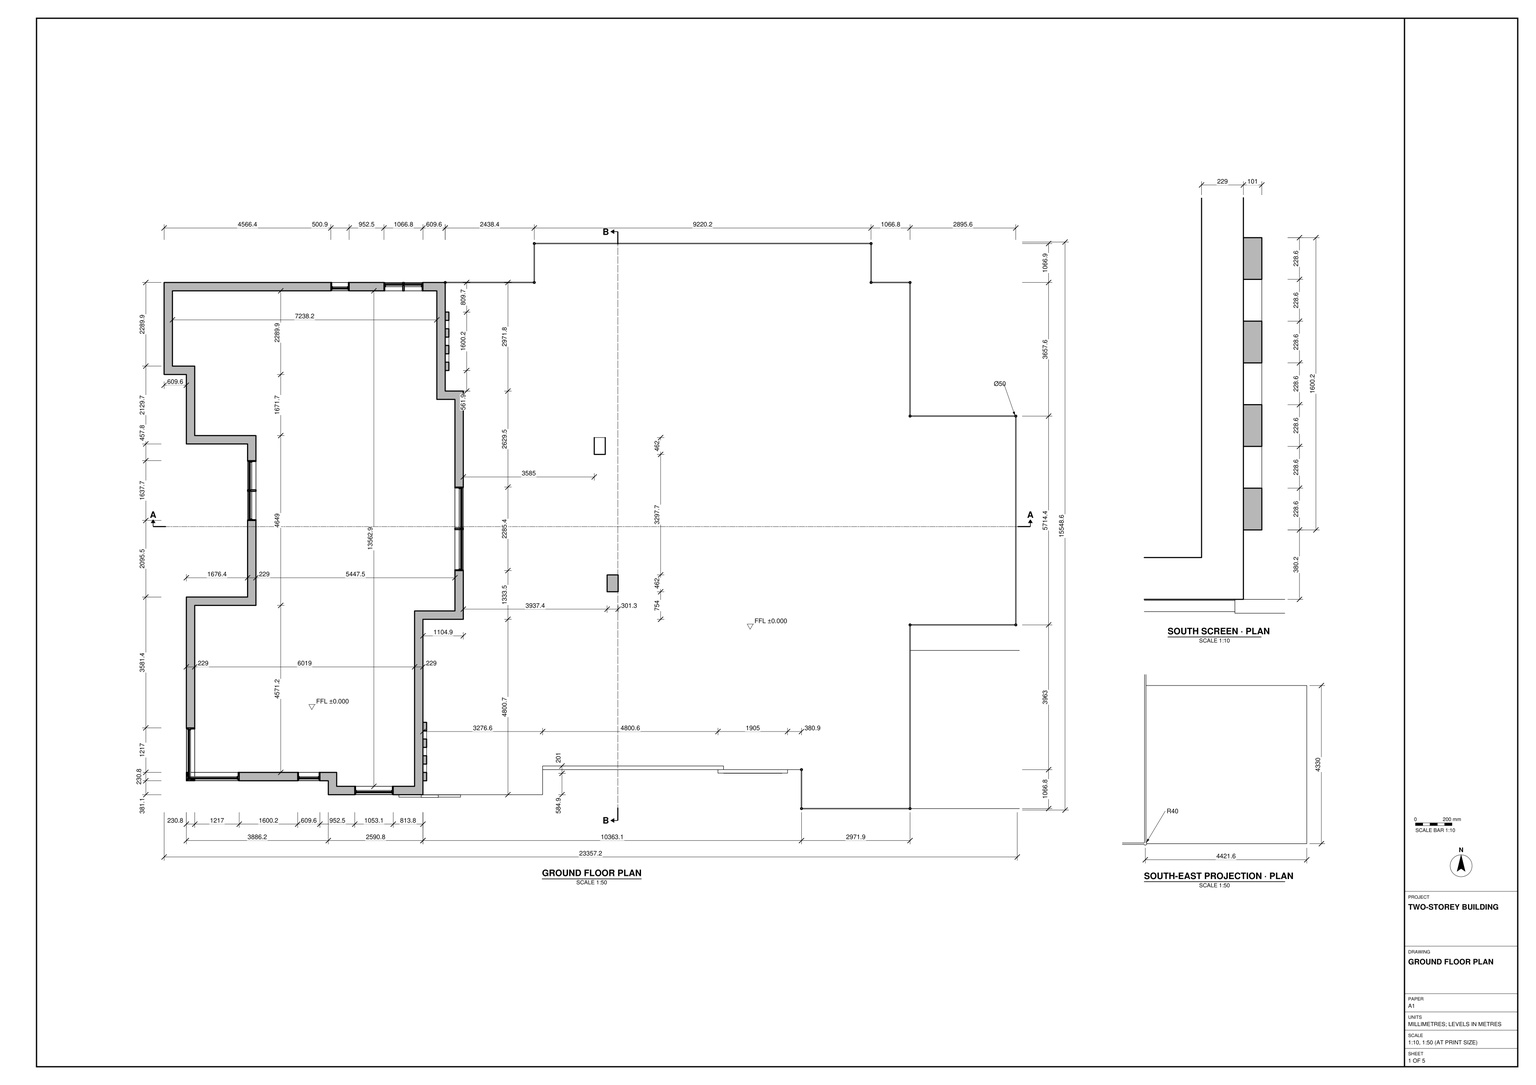
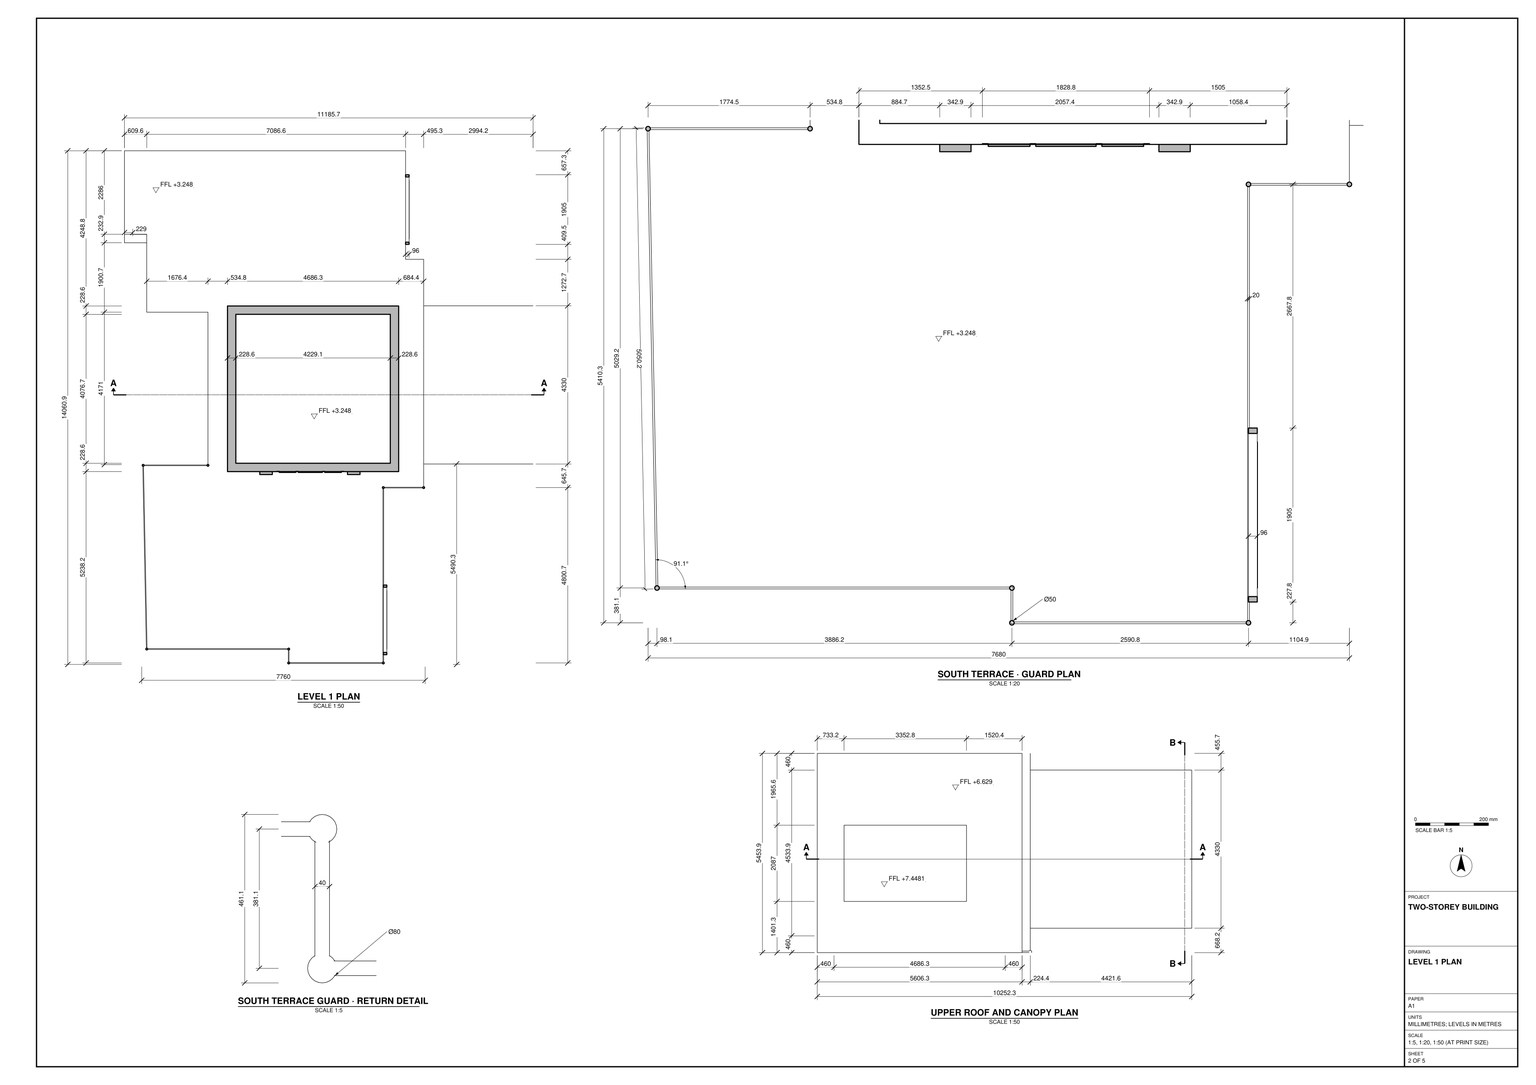
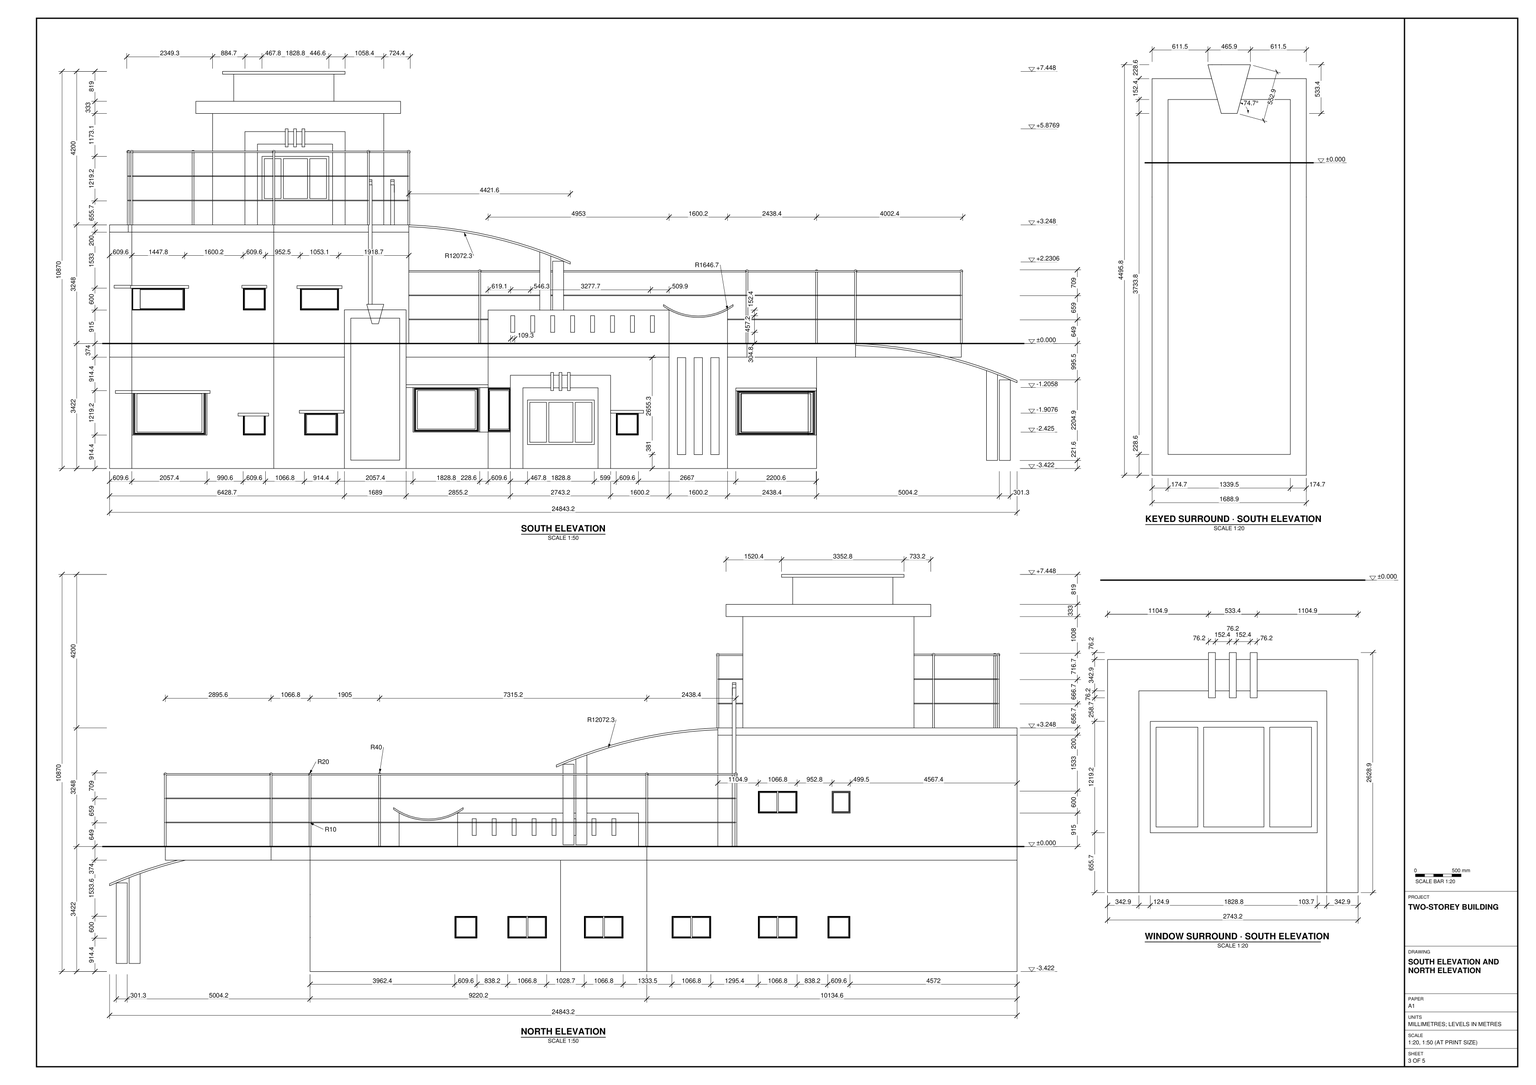
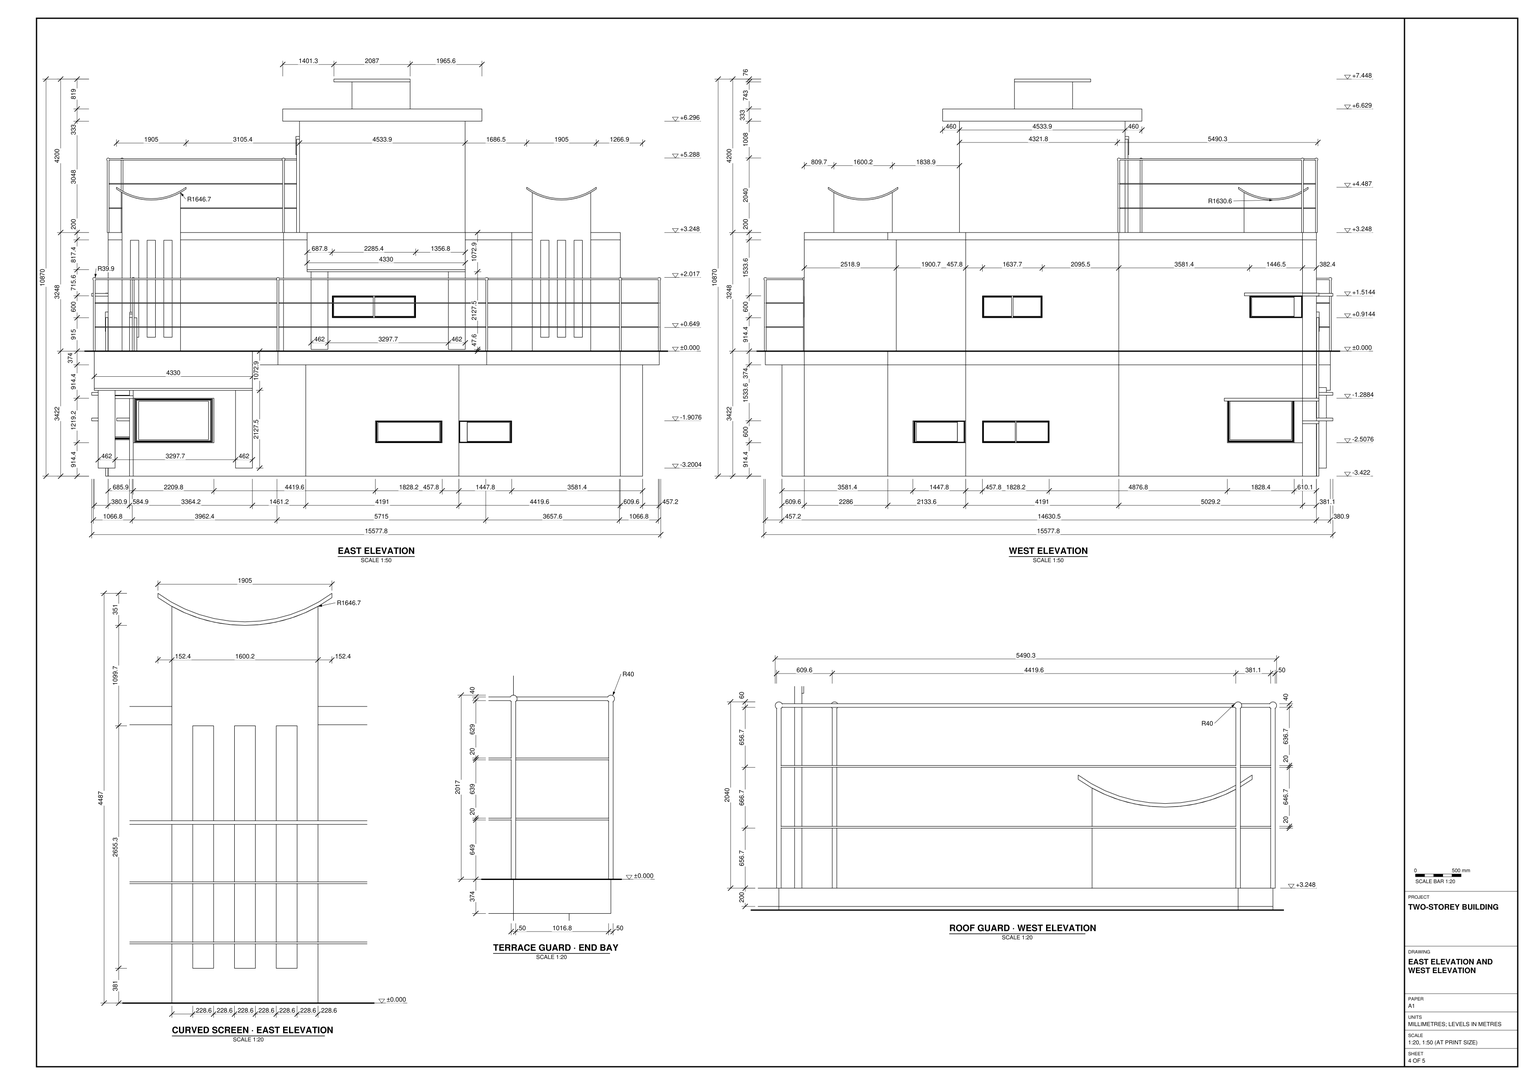
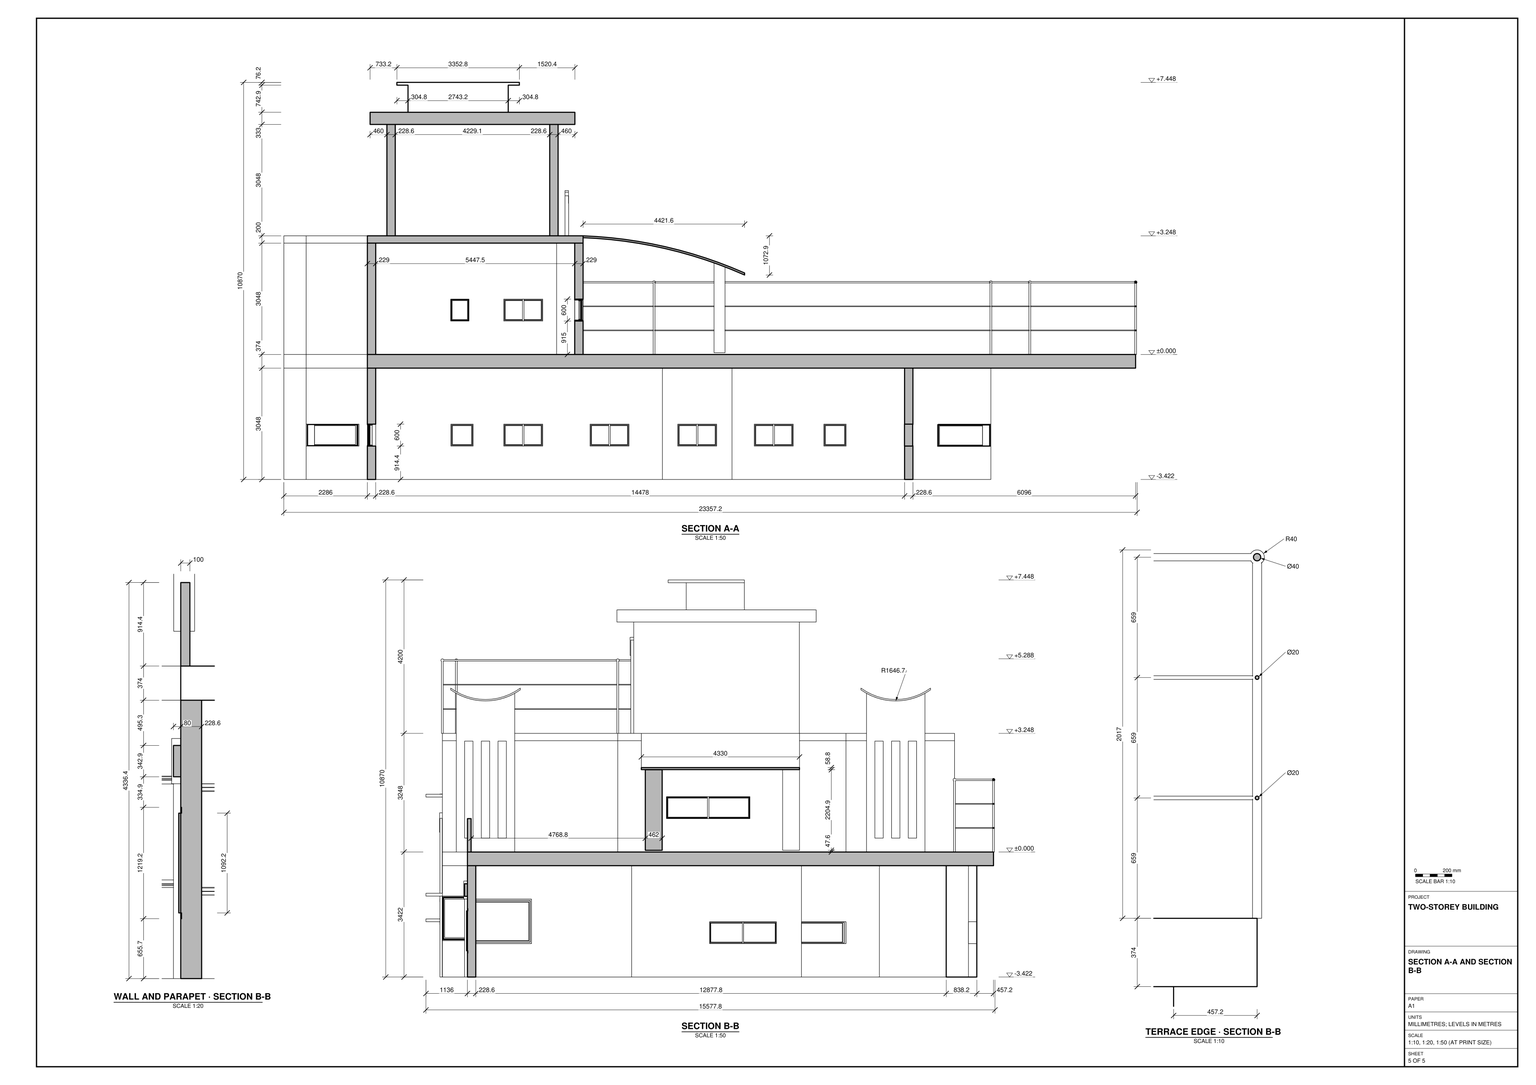
Build the building shown in task_files/diagram_01.pdf in SketchUp. Work in millimetres. The overall extents, including roof edges and canopy projections, are 24843.2 mm along X, 15577.7 mm along Y and 10870.1 mm along Z. Set the ground-floor datum at 0 mm and Level 1 at +3248 mm. Include the part of the building below the ground-floor datum shown in the elevations.

Trace the stepped ground-floor enclosure on the west side of the plan, using the drawn wall thickness of 229 mm. Above it, form the smaller rectangular enclosure with 228.6 mm walls. Follow the slab outlines so that the terraces retain their recesses and projecting corners. Model the terrace guards with horizontal rails, posts and the south return. Give the upper enclosure its overhanging flat roof and smaller raised cap. Follow the elevation profiles for the curved canopies and place their supports as drawn.

Set the window openings and frame divisions from the elevations. Include the tall keyed surround, the framed south windows and the vertical screen detail. Keep shell elements and each furniture or joinery piece shown in separate groups or components, and use components for repeated parts. Decor and loose items may be any suitable library components. Save one SketchUp model as output_files/two_storey_building_stepped_terraces_and_curved_canopies.skp.

# SketchUp Ruby script. Lengths in millimetres.
U = 1.mm
M = Sketchup.active_model
def pt(a) = Geom::Point3d.new(a.map { |v| v * U })
def face(e, loops, mat)
  f = e.add_face(loops[0].map { |a| pt(a) })
  loops[1..].each { |l| e.add_face(l.map { |a| pt(a) }).erase! }
  f.material = f.back_material = mat if mat
  f
end
# faces: each face lists its corners as indices into pts; further lists are holes
def faces(e, pts, list, mat = nil) = list.each { |f| face(e, (f[0].is_a?(Array) ? f : [f]).map { |l| l.map { |i| pts[i] } }, mat) }
# xy, xz, yz: faces in a plane at the given z, y or x. An outline is a flat list of corners, or four numbers for a rectangle; further outlines are holes
def ring(l) = l.size == 4 ? [[l[0], l[1]], [l[2], l[1]], [l[2], l[3]], [l[0], l[3]]] : l.each_slice(2).to_a
def flat(e, list, mat, &to3) = list.each { |f| face(e, (f[0].is_a?(Array) ? f : [f]).map { |l| ring(l).map { |u, v| to3.(u, v) } }, mat) }
def xy(e, z, list, mat = nil) = flat(e, list, mat) { |x, y| [x, y, z] }
def xz(e, y, list, mat = nil) = flat(e, list, mat) { |x, z| [x, y, z] }
def yz(e, x, list, mat = nil) = flat(e, list, mat) { |y, z| [x, y, z] }
def lines(e, pts, list) = list.each { |a, b| e.add_line(pt(pts[a]), pt(pts[b])) }
# prism: a flat outline (further loops are holes) pulled along v
def prism(e, loops, v, mat = nil)
  f = face(e, loops, mat); d = Geom::Vector3d.new(v.map { |x| x * U })
  f.pushpull(f.normal.samedirection?(d) ? d.length : -d.length)
end
def box(e, o, s, mat = nil) = prism(e, [[o, [o[0] + s[0], o[1], o[2]], [o[0] + s[0], o[1] + s[1], o[2]], [o[0], o[1] + s[1], o[2]]]], [0, 0, s[2]], mat)
def at(x, y, z, deg = 0) = Geom::Transformation.translation(pt([x, y, z])) * Geom::Transformation.rotation(ORIGIN, Z_AXIS, deg.degrees)
def axes(o, x, y, z) = Geom::Transformation.new([*x, 0, *y, 0, *z, 0, *pt(o).to_a, 1])
def part(name) = M.definitions.add(name)
# library, detail: a bought-in or finely detailed component or shape, given as its bounding box
def library(name, o, s) = part(name).tap { |d| box(d.entities, o, s) }
def detail(e, o, s) = box(e.add_group.entities, o, s)
def put(e, d, t, mat = nil) = e.add_instance(d, t).tap { |i| i.material = mat if mat }
def group(e, t, mat = nil) = e.add_group.tap { |g| g.transformation = t; g.material = mat if mat }.entities
root = M.entities
M.materials.add("[0012_Bisque]").color = [255, 228, 196]
M.materials.add("[Stone Marble]").color = [143, 138, 136]
M.materials.add("[Wood Cherry Original]").color = [152, 86, 42]
c1 = part("Difference\#1")
xy(c1.entities,0,[[[4495.8,0,4495.8,381.1,609.6,381.1,609.6,5410.3,2286,5410.3,2286,9601.3,609.6,9601.3,609.6,11734.9,0,11734.9,0,14020.9,10134.6,14020.9,10134.6,14630.5,12496.8,14630.5,12496.8,14020.9,19354.8,14020.9,19354.8,9601.3,17221.2,9601.3,17221.2,5410.3,19354.8,5410.3,19354.8,685.9,10363.2,685.9,10363.2,0],[4724.4,228.6,10134.6,228.6,10134.6,914.5,19126.2,914.5,19126.2,5181.7,16992.6,5181.7,16992.6,9829.9,19126.2,9829.9,19126.2,13792.3,12268.2,13792.3,12268.2,14401.9,10363.2,14401.9,10363.2,13792.3,228.6,13792.3,228.6,11963.5,838.2,11963.5,838.2,9829.9,2514.6,9829.9,2514.6,5181.7,838.2,5181.7,838.2,609.7,4724.4,609.7]]])
xy(c1.entities,914.4,[[5334,0,6248.4,228.6],[609.6,381.1,2667,381.1,2667,609.7,838.2,609.7,838.2,2438.5,609.6,2438.5],[3657.6,381.1,4267.2,609.7],[13868.4,685.9,14478,914.5],[17145,685.9,19354.8,685.9,19354.8,2895.7,19126.2,2895.7,19126.2,914.5,17145,914.5],
  [2286,7315.3,2514.6,9143.5],[16992.6,7315.3,17221.2,9143.5],[609.6,9601.3,2057.4,9601.3,2057.4,9829.9,838.2,9829.9,838.2,11049.1,609.6,11049.1],[17907,9601.3,19354.8,9601.3,19354.8,11049.1,19126.2,11049.1,19126.2,9829.9,17907,9829.9],[4572,13792.3,5181.6,14020.9],
  [6019.8,13792.3,7086.6,14020.9],[8382,13792.3,9448.8,14020.9],[12877.8,13792.3,13944.6,14020.9],[14782.8,13792.3,15392.4,14020.9],[10782.3,14401.9,11849.1,14630.5]])
xy(c1.entities,997,[[8305.8,0,10363.2,0,10363.2,685.9,10972.8,685.9,10972.8,914.5,10134.6,914.5,10134.6,228.6,8305.8,228.6]])
xy(c1.entities,1514.4,[[5334,0,6248.4,228.6],[3657.6,381.1,4267.2,609.7],[13868.4,685.9,14478,914.5],[2286,7315.3,2514.6,9143.5],[16992.6,7315.3,17221.2,9143.5],
  [609.6,9601.3,609.6,11049.1,838.2,11049.1,838.2,9829.9,2057.4,9829.9,2057.4,9601.3],[17907,9601.3,17907,9829.9,19126.2,9829.9,19126.2,11049.1,19354.8,11049.1,19354.8,9601.3],[4572,13792.3,5181.6,14020.9],[6019.8,13792.3,7086.6,14020.9],[8382,13792.3,9448.8,14020.9],
  [12877.8,13792.3,13944.6,14020.9],[14782.8,13792.3,15392.4,14020.9],[10782.3,14401.9,11849.1,14630.5]])
xy(c1.entities,2133.6,[[609.6,381.1,609.6,2438.5,838.2,2438.5,838.2,609.7,2667,609.7,2667,381.1],[17145,685.9,17145,914.5,19126.2,914.5,19126.2,2895.7,19354.8,2895.7,19354.8,685.9]])
xy(c1.entities,2216.2,[[8305.8,0,8305.8,228.6,10134.6,228.6,10134.6,914.5,10972.8,914.5,10972.8,685.9,10363.2,685.9,10363.2,0]])
xy(c1.entities,3048,[[[4495.8,0,10363.2,0,10363.2,685.9,19354.8,685.9,19354.8,5410.3,17221.2,5410.3,17221.2,9601.3,19354.8,9601.3,19354.8,14020.9,12496.8,14020.9,12496.8,14630.5,10134.6,14630.5,10134.6,14020.9,0,14020.9,0,11734.9,609.6,11734.9,609.6,9601.3,2286,9601.3,2286,5410.3,609.6,5410.3,609.6,381.1,4495.8,381.1],[4724.4,228.6,4724.4,609.7,838.2,609.7,838.2,5181.7,2514.6,5181.7,2514.6,9829.9,838.2,9829.9,838.2,11963.5,228.6,11963.5,228.6,13792.3,10363.2,13792.3,10363.2,14401.9,12268.2,14401.9,12268.2,13792.3,19126.2,13792.3,19126.2,9829.9,16992.6,9829.9,16992.6,5181.7,19126.2,5181.7,19126.2,914.5,10134.6,914.5,10134.6,228.6]]])
xz(c1.entities,0,[[[4495.8,0,10363.2,0,10363.2,997,8305.8,997,8305.8,2216.2,10363.2,2216.2,10363.2,3048,4495.8,3048],[5334,914.4,6248.4,1514.4]]])
xz(c1.entities,228.6,[[[4724.4,0,4724.4,3048,10134.6,3048,10134.6,2216.2,8305.8,2216.2,8305.8,997,10134.6,997,10134.6,0],[5334,914.4,6248.4,1514.4]]])
xz(c1.entities,381.1,[[[609.6,0,4495.8,0,4495.8,3048,609.6,3048,609.6,2133.6,2667,2133.6,2667,914.4,609.6,914.4],[3657.6,914.4,4267.2,1514.4]]])
xz(c1.entities,609.7,[[[838.2,0,838.2,914.4,2667,914.4,2667,2133.6,838.2,2133.6,838.2,3048,4724.4,3048,4724.4,0],[3657.6,914.4,4267.2,1514.4]]])
xz(c1.entities,685.9,[[[10363.2,0,19354.8,0,19354.8,914.4,17145,914.4,17145,2133.6,19354.8,2133.6,19354.8,3048,10363.2,3048,10363.2,2216.2,10972.8,2216.2,10972.8,997,10363.2,997],[13868.4,914.4,14478,1514.4]]])
xz(c1.entities,914.5,[[[10134.6,0,10134.6,997,10972.8,997,10972.8,2216.2,10134.6,2216.2,10134.6,3048,19126.2,3048,19126.2,2133.6,17145,2133.6,17145,914.4,19126.2,914.4,19126.2,0],[13868.4,914.4,14478,1514.4]]])
xz(c1.entities,2438.5,[[609.6,914.4,838.2,2133.6]])
xz(c1.entities,2895.7,[[19126.2,914.4,19354.8,2133.6]])
xz(c1.entities,5181.7,[[838.2,0,2514.6,3048],[16992.6,0,19126.2,3048]])
xz(c1.entities,5410.3,[[609.6,0,2286,3048],[17221.2,0,19354.8,3048]])
xz(c1.entities,7315.3,[[2286,914.4,2514.6,1514.4],[16992.6,914.4,17221.2,1514.4]])
xz(c1.entities,9143.5,[[2286,914.4,2514.6,1514.4],[16992.6,914.4,17221.2,1514.4]])
xz(c1.entities,9601.3,[[609.6,0,2286,0,2286,3048,609.6,3048,609.6,1514.4,2057.4,1514.4,2057.4,914.4,609.6,914.4],[17221.2,0,19354.8,0,19354.8,914.4,17907,914.4,17907,1514.4,19354.8,1514.4,19354.8,3048,17221.2,3048]])
xz(c1.entities,9829.9,[[838.2,0,838.2,914.4,2057.4,914.4,2057.4,1514.4,838.2,1514.4,838.2,3048,2514.6,3048,2514.6,0],[16992.6,0,16992.6,3048,19126.2,3048,19126.2,1514.4,17907,1514.4,17907,914.4,19126.2,914.4,19126.2,0]])
xz(c1.entities,11049.1,[[609.6,914.4,838.2,1514.4],[19126.2,914.4,19354.8,1514.4]])
xz(c1.entities,11734.9,[[0,0,609.6,3048]])
xz(c1.entities,11963.5,[[228.6,0,838.2,3048]])
xz(c1.entities,13792.3,[[[228.6,0,10363.2,3048],[8382,914.4,9448.8,1514.4],[6019.8,914.4,7086.6,1514.4],[4572,914.4,5181.6,1514.4]],[[12268.2,0,19126.2,3048],[12877.8,914.4,13944.6,1514.4],[14782.8,914.4,15392.4,1514.4]]])
xz(c1.entities,14020.9,[[[0,0,10134.6,3048],[8382,914.4,9448.8,1514.4],[6019.8,914.4,7086.6,1514.4],[4572,914.4,5181.6,1514.4]],[[12496.8,0,19354.8,3048],[12877.8,914.4,13944.6,1514.4],[14782.8,914.4,15392.4,1514.4]]])
xz(c1.entities,14401.9,[[[10363.2,0,12268.2,3048],[10782.3,914.4,11849.1,1514.4]]])
xz(c1.entities,14630.5,[[[10134.6,0,12496.8,3048],[10782.3,914.4,11849.1,1514.4]]])
yz(c1.entities,0,[[11734.9,0,14020.9,3048]])
yz(c1.entities,228.6,[[11963.5,0,13792.3,3048]])
yz(c1.entities,609.6,[[381.1,0,381.1,914.4,2438.5,914.4,2438.5,2133.6,381.1,2133.6,381.1,3048,5410.3,3048,5410.3,0],[9601.3,0,9601.3,914.4,11049.1,914.4,11049.1,1514.4,9601.3,1514.4,9601.3,3048,11734.9,3048,11734.9,0]])
yz(c1.entities,838.2,[[609.7,0,5181.7,0,5181.7,3048,609.7,3048,609.7,2133.6,2438.5,2133.6,2438.5,914.4,609.7,914.4],[9829.9,0,11963.5,0,11963.5,3048,9829.9,3048,9829.9,1514.4,11049.1,1514.4,11049.1,914.4,9829.9,914.4]])
yz(c1.entities,2057.4,[[9601.3,914.4,9829.9,1514.4]])
yz(c1.entities,2286,[[[5410.3,0,9601.3,3048],[7315.3,914.4,9143.5,1514.4]]])
yz(c1.entities,2514.6,[[[5181.7,0,9829.9,3048],[7315.3,914.4,9143.5,1514.4]]])
yz(c1.entities,2667,[[381.1,914.4,609.7,2133.6]])
yz(c1.entities,3657.6,[[381.1,914.4,609.7,1514.4]])
yz(c1.entities,4267.2,[[381.1,914.4,609.7,1514.4]])
yz(c1.entities,4495.8,[[0,0,381.1,3048]])
yz(c1.entities,4572,[[13792.3,914.4,14020.9,1514.4]])
yz(c1.entities,4724.4,[[228.6,0,609.7,3048]])
yz(c1.entities,5181.6,[[13792.3,914.4,14020.9,1514.4]])
yz(c1.entities,5334,[[0,914.4,228.6,1514.4]])
yz(c1.entities,6019.8,[[13792.3,914.4,14020.9,1514.4]])
yz(c1.entities,6248.4,[[0,914.4,228.6,1514.4]])
yz(c1.entities,7086.6,[[13792.3,914.4,14020.9,1514.4]])
yz(c1.entities,8305.8,[[0,997,228.6,2216.2]])
yz(c1.entities,8382,[[13792.3,914.4,14020.9,1514.4]])
yz(c1.entities,9448.8,[[13792.3,914.4,14020.9,1514.4]])
yz(c1.entities,10134.6,[[228.6,0,914.5,997],[14020.9,0,14630.5,3048],[228.6,2216.2,914.5,3048]])
yz(c1.entities,10363.2,[[0,0,685.9,997],[13792.3,0,14401.9,3048],[0,2216.2,685.9,3048]])
yz(c1.entities,10782.3,[[14401.9,914.4,14630.5,1514.4]])
yz(c1.entities,10972.8,[[685.9,997,914.5,2216.2]])
yz(c1.entities,11849.1,[[14401.9,914.4,14630.5,1514.4]])
yz(c1.entities,12268.2,[[13792.3,0,14401.9,3048]])
yz(c1.entities,12496.8,[[14020.9,0,14630.5,3048]])
yz(c1.entities,12877.8,[[13792.3,914.4,14020.9,1514.4]])
yz(c1.entities,13868.4,[[685.9,914.4,914.5,1514.4]])
yz(c1.entities,13944.6,[[13792.3,914.4,14020.9,1514.4]])
yz(c1.entities,14478,[[685.9,914.4,914.5,1514.4]])
yz(c1.entities,14782.8,[[13792.3,914.4,14020.9,1514.4]])
yz(c1.entities,15392.4,[[13792.3,914.4,14020.9,1514.4]])
yz(c1.entities,16992.6,[[[5181.7,0,9829.9,3048],[7315.3,914.4,9143.5,1514.4]]])
yz(c1.entities,17145,[[685.9,914.4,914.5,2133.6]])
yz(c1.entities,17221.2,[[[5410.3,0,9601.3,3048],[7315.3,914.4,9143.5,1514.4]]])
yz(c1.entities,17907,[[9601.3,914.4,9829.9,1514.4]])
yz(c1.entities,19126.2,[[914.5,0,914.5,914.4,2895.7,914.4,2895.7,2133.6,914.5,2133.6,914.5,3048,5181.7,3048,5181.7,0],[9829.9,0,9829.9,914.4,11049.1,914.4,11049.1,1514.4,9829.9,1514.4,9829.9,3048,13792.3,3048,13792.3,0]])
yz(c1.entities,19354.8,[[685.9,0,5410.3,0,5410.3,3048,685.9,3048,685.9,2133.6,2895.7,2133.6,2895.7,914.4,685.9,914.4],[9601.3,0,14020.9,0,14020.9,3048,9601.3,3048,9601.3,1514.4,11049.1,1514.4,11049.1,914.4,9601.3,914.4]])
c2 = part("Group\#19")
box(c2.entities,[-87,0,0],[1590,450,77])
c3 = part("Group\#20")
g1 = group(c3.entities,at(0,-450,0))
box(g1,[0,0,0],[2141,450,77])
c4 = library("Group\#35",[0,0,0],[609.6,230.8,600])
c5 = part("Difference\#7")
xy(c5.entities,0,[[[4495.8,0,4495.8,381.1,609.6,381.1,609.6,5410.3,2286,5410.3,2286,9601.3,609.6,9601.3,609.6,11502,0,11502,0,14020.9,7696.2,14020.9,7696.2,11049.1,8191.5,11049.1,8191.5,4800.7,7086.6,4800.7,7086.6,0],[4724.8,229,6857.6,229,6857.6,5029.7,7962.5,5029.7,7962.5,10820.1,7467.2,10820.1,7467.2,13791.9,229,13791.9,229,11731,838.6,11731,838.6,9830.3,2515,9830.3,2515,5181.3,838.6,5181.3,838.6,610.1,4724.8,610.1]]])
xy(c5.entities,914.4,[[609.6,381.1,2057.4,381.1,2057.4,610.1,838.6,610.1,838.6,1828.9,609.6,1828.9]])
xy(c5.entities,915,[[5219.7,0,6272.8,229],[3657.6,381.1,4267.2,610.1],[7962.5,6134.2,8191.5,8419.6],[2286,7505.8,2515,9143.5],[4566.4,13791.9,5067.3,14020.9],
  [6019.8,13791.9,7086.6,14020.9]])
xy(c5.entities,1514.4,[[609.6,381.1,609.6,1828.9,838.6,1828.9,838.6,610.1,2057.4,610.1,2057.4,381.1]])
xy(c5.entities,1515,[[5219.7,0,6272.8,229],[3657.6,381.1,4267.2,610.1],[7962.5,6134.2,8191.5,8419.6],[2286,7505.8,2515,9143.5],[4566.4,13791.9,5067.3,14020.9],
  [6019.8,13791.9,7086.6,14020.9]])
xy(c5.entities,3048,[[[4495.8,0,7086.6,0,7086.6,4800.7,8191.5,4800.7,8191.5,11049.1,7696.2,11049.1,7696.2,14020.9,0,14020.9,0,11502,609.6,11502,609.6,9601.3,2286,9601.3,2286,5410.3,609.6,5410.3,609.6,381.1,4495.8,381.1],[4724.8,229,4724.8,610.1,838.6,610.1,838.6,5181.3,2515,5181.3,2515,9830.3,838.6,9830.3,838.6,11731,229,11731,229,13791.9,7467.2,13791.9,7467.2,10820.1,7962.5,10820.1,7962.5,5029.7,6857.6,5029.7,6857.6,229]]])
xz(c5.entities,0,[[[4495.8,0,7086.6,3048],[5219.7,915,6272.8,1515]]])
xz(c5.entities,229,[[[4724.8,0,6857.6,3048],[5219.7,915,6272.8,1515]]])
xz(c5.entities,381.1,[[[609.6,0,4495.8,0,4495.8,3048,609.6,3048,609.6,1514.4,2057.4,1514.4,2057.4,914.4,609.6,914.4],[3657.6,915,4267.2,1515]]])
xz(c5.entities,610.1,[[[838.6,0,838.6,914.4,2057.4,914.4,2057.4,1514.4,838.6,1514.4,838.6,3048,4724.8,3048,4724.8,0],[3657.6,915,4267.2,1515]]])
xz(c5.entities,1828.9,[[609.6,914.4,838.6,1514.4]])
xz(c5.entities,4800.7,[[7086.6,0,8191.5,3048]])
xz(c5.entities,5029.7,[[6857.6,0,7962.5,3048]])
xz(c5.entities,5181.3,[[838.6,0,2515,3048]])
xz(c5.entities,5410.3,[[609.6,0,2286,3048]])
xz(c5.entities,6134.2,[[7962.5,915,8191.5,1515]])
xz(c5.entities,7505.8,[[2286,915,2515,1515]])
xz(c5.entities,8419.6,[[7962.5,915,8191.5,1515]])
xz(c5.entities,9143.5,[[2286,915,2515,1515]])
xz(c5.entities,9601.3,[[609.6,0,2286,3048]])
xz(c5.entities,9830.3,[[838.6,0,2515,3048]])
xz(c5.entities,10820.1,[[7467.2,0,7962.5,3048]])
xz(c5.entities,11049.1,[[7696.2,0,8191.5,3048]])
xz(c5.entities,11502,[[0,0,609.6,3048]])
xz(c5.entities,11731,[[229,0,838.6,3048]])
xz(c5.entities,13791.9,[[[229,0,7467.2,3048],[6019.8,915,7086.6,1515],[4566.4,915,5067.3,1515]]])
xz(c5.entities,14020.9,[[[0,0,7696.2,3048],[6019.8,915,7086.6,1515],[4566.4,915,5067.3,1515]]])
yz(c5.entities,0,[[11502,0,14020.9,3048]])
yz(c5.entities,229,[[11731,0,13791.9,3048]])
yz(c5.entities,609.6,[[381.1,0,381.1,914.4,1828.9,914.4,1828.9,1514.4,381.1,1514.4,381.1,3048,5410.3,3048,5410.3,0],[9601.3,0,11502,3048]])
yz(c5.entities,838.6,[[610.1,0,5181.3,0,5181.3,3048,610.1,3048,610.1,1514.4,1828.9,1514.4,1828.9,914.4,610.1,914.4],[9830.3,0,11731,3048]])
yz(c5.entities,2057.4,[[381.1,914.4,610.1,1514.4]])
yz(c5.entities,2286,[[[5410.3,0,9601.3,3048],[7505.8,915,9143.5,1515]]])
yz(c5.entities,2515,[[[5181.3,0,9830.3,3048],[7505.8,915,9143.5,1515]]])
yz(c5.entities,3657.6,[[381.1,915,610.1,1515]])
yz(c5.entities,4267.2,[[381.1,915,610.1,1515]])
yz(c5.entities,4495.8,[[0,0,381.1,3048]])
yz(c5.entities,4566.4,[[13791.9,915,14020.9,1515]])
yz(c5.entities,4724.8,[[229,0,610.1,3048]])
yz(c5.entities,5067.3,[[13791.9,915,14020.9,1515]])
yz(c5.entities,5219.7,[[0,915,229,1515]])
yz(c5.entities,6019.8,[[13791.9,915,14020.9,1515]])
yz(c5.entities,6272.8,[[0,915,229,1515]])
yz(c5.entities,6857.6,[[229,0,5029.7,3048]])
yz(c5.entities,7086.6,[[0,0,4800.7,3048],[13791.9,915,14020.9,1515]])
yz(c5.entities,7467.2,[[10820.1,0,13791.9,3048]])
yz(c5.entities,7696.2,[[11049.1,0,14020.9,3048]])
yz(c5.entities,7962.5,[[[5029.7,0,10820.1,3048],[6134.2,915,8419.6,1515]]])
yz(c5.entities,8191.5,[[[4800.7,0,11049.1,3048],[6134.2,915,8419.6,1515]]])
c6 = library("Group\#15",[0,0,0],[230.8,2285.4,600])
c7 = part("Difference\#6")
put(c7.entities,c5,at(0,0,0))
put(c7.entities,c6,at(7960.7,6134.2,915))
put(c7.entities,c6,axes([2417.6,9143.5,-2507.6],[-0.57,0,0],[0,-0.79995,0],[0,0,1]))
c8 = library("Group\#13",[0,0,0],[1066.8,230.8,600])
c9 = part("Difference\#5")
put(c9.entities,c7,at(0,0,0))
put(c9.entities,c8,at(6019.8,13790,915))
put(c9.entities,c8,at(8382,13790,-2507.6))
put(c9.entities,c8,at(6019.8,13790,-2507.6))
put(c9.entities,c8,at(10782.3,14399.6,-2507.6))
put(c9.entities,c8,at(12877.8,13790,-2507.6))
c10 = library("Group\#11",[0,0,0],[500.9,230.8,600])
c11 = part("Difference\#4")
put(c11.entities,c9,at(0,0,0))
put(c11.entities,c10,at(5067.3,14022.7,915,180))
c12 = library("Group\#9",[0,0,0],[230.8,1637.7,600])
c13 = part("Difference\#3")
put(c13.entities,c11,at(0,0,0))
put(c13.entities,c12,at(2286,7505.8,915))
c14 = library("Group\#7",[0,0,0],[1053.1,230.8,600])
c15 = part("Difference\#2")
put(c15.entities,c13,at(0,0,0))
put(c15.entities,c14,at(5219.7,0,915))
put(c15.entities,c14,axes([610.9,381.1,914.4],[1.3736,0,0],[0,1,0],[0,0,1]))
put(c15.entities,c14,axes([609.6,1828.9,914.4],[0,-1.3736,0],[1,0,0],[0,0,1]))
put(c15.entities,c14,axes([609.6,2438.5,-2507.6],[0,-1.73622,0],[1,0,0],[0,0,2.032]))
put(c15.entities,c14,axes([17893.3,9601.3,-2517.6],[1.37481,0,0],[0,1,0],[0,0,1]))
put(c15.entities,c14,axes([19354.8,9601.3,-2507.6],[0,1.37481,0],[-1,0,0],[0,0,1]))
put(c15.entities,c14,axes([17221.2,7315.3,-2507.6],[0,1.73603,0],[-1,0,0],[0,0,1]))
c16 = library("Group\#16",[0,0,0],[609.6,230.8,600])
c17 = library("Group\#44",[0,0,0],[2743.2,2628.9,100])
c18 = part("Group\#45")
xy(c18.entities,0,[[[0,0,1828.8,1219.2],[584.2,63.5,1244.6,1155.7],[63.5,63.5,520.7,1155.7],[1308.1,63.5,1765.3,1155.7]]])
xy(c18.entities,8,[[[0,0,1828.8,1219.2],[584.2,63.5,1244.6,1155.7],[63.5,63.5,520.7,1155.7],[1308.1,63.5,1765.3,1155.7]]])
xy(c18.entities,30,[[63.5,63.5,520.7,1155.7],[584.2,63.5,1244.6,1155.7],[1308.1,63.5,1765.3,1155.7]])
xz(c18.entities,0,[[0,0,1828.8,8]])
xz(c18.entities,63.5,[[63.5,8,520.7,30],[584.2,8,1244.6,30],[1308.1,8,1765.3,30]])
xz(c18.entities,1155.7,[[63.5,8,520.7,30],[584.2,8,1244.6,30],[1308.1,8,1765.3,30]])
xz(c18.entities,1219.2,[[0,0,1828.8,8]])
yz(c18.entities,0,[[0,0,1219.2,8]])
yz(c18.entities,63.5,[[63.5,8,1155.7,30]])
yz(c18.entities,520.7,[[63.5,8,1155.7,30]])
yz(c18.entities,584.2,[[63.5,8,1155.7,30]])
yz(c18.entities,1244.6,[[63.5,8,1155.7,30]])
yz(c18.entities,1308.1,[[63.5,8,1155.7,30]])
yz(c18.entities,1765.3,[[63.5,8,1155.7,30]])
yz(c18.entities,1828.8,[[0,0,1219.2,8]])
p = [[520.7,1155.7,0],[520.7,1155.7,8],[63.5,1155.7,0],[63.5,1155.7,8],[520.7,63.5,0],[520.7,63.5,8],
  [63.5,63.5,0],[63.5,63.5,8],[584.2,1155.7,0],[584.2,1155.7,8],[584.2,63.5,0],[584.2,63.5,8],
  [1244.6,1155.7,0],[1244.6,1155.7,8],[1244.6,63.5,0],[1244.6,63.5,8],[1308.1,1155.7,0],[1308.1,1155.7,8],
  [1308.1,63.5,0],[1308.1,63.5,8],[1765.3,1155.7,0],[1765.3,1155.7,8],[1765.3,63.5,0],[1765.3,63.5,8]]
lines(c18.entities,p,[[0,1],[2,3],[4,5],[6,7],[8,9],[10,11],[12,13],[14,15],[16,17],[18,19],[20,21],[22,23]])
c19 = library("Group\#48",[0,0,0],[1905,4487,101])
c20 = library("Group\#51",[0,0,0],[4421.6,3200.4,4330])
c21 = part("Group\#52")
box(c21.entities,[0,0,0],[301.3,462,2204.9])
c22 = library("Group\#58",[0,0,0],[2743.2,2628.9,100])
c23 = library("Ploe\#1",[10952.3,37271.5,6670],[80,80,2040])
c24 = part("Group73\#1")
put(c24.entities,c23,at(0,0,0))
put(c24.entities,c23,at(-1774.5,0,0))
put(c24.entities,c23,at(-1676.4,-5029.2,0))
put(c24.entities,c23,at(2209.8,-5029.2,0))
put(c24.entities,c23,at(2209.8,-5410.3,0))
put(c24.entities,c23,at(4800.6,-5410.3,0))
put(c24.entities,c23,at(4800.6,-609.6,0))
put(c24.entities,c23,at(5905.5,-609.6,0))
c25 = library("Group74\#1",[9197.4,31881.2,7326.7],[7700.4,5450.3,1363.3])
c26 = library("Group78\#1",[16402.5,31500.3,4071],[15641,15508.6,1348])
c27 = library("Ploe\#2",[26116.1,32547.1,3422],[80,80,2017])
c28 = part("Group77\#1")
put(c28.entities,c27,at(0,0,0))
put(c28.entities,c27,at(0,-1066.8,0))
put(c28.entities,c27,at(2971.8,-1066.8,0))
put(c28.entities,c27,at(2971.8,3962.4,0))
put(c28.entities,c27,at(5867.4,3962.4,0))
put(c28.entities,c27,at(5867.4,9677.4,0))
put(c28.entities,c27,at(2971.8,9677.4,0))
put(c28.entities,c27,at(2971.8,13335,0))
put(c28.entities,c27,at(1905,13335,0))
put(c28.entities,c27,at(1905,14401.8,0))
put(c28.entities,c27,at(-7315.2,14401.8,0))
put(c28.entities,c27,at(-7315.2,13335,0))
put(c28.entities,c27,at(-9753.6,13335,0))
put(root,c1,at(0,450,0))
g2 = group(root,at(0,69.1,3048))
prism(g2,[[[4495.8,762,0],[609.6,762,0],[609.6,5791.2,0],[2286,5791.2,0],[2286,9982.2,0],[609.6,9982.2,0],[609.6,12115.8,0],[0,12115.8,0],[0,14401.8,0],[10134.6,14401.8,0],[10134.6,15468.6,0],[19354.8,15468.6,0],[19354.8,14401.8,0],[20421.6,14401.8,0],[20421.6,10744.2,0],[23317.2,10744.2,0],[23317.2,5029.2,0],[20421.6,5029.2,0],[20421.6,0,0],[17449.8,0,0],[17449.8,1066.8,0],[10363.2,1066.8,0],[10363.2,380.9,0],[4495.8,380.9,0]]],[0,0,374])
g3 = group(root,at(5130.2,450,4927))
g4 = group(g3,at(0,-450,0))
box(g4,[0,0,0],[1232,450,77])
g5 = group(root,at(3589,831.1,4936.7))
g6 = group(g5,at(0,-356.9,0))
box(g6,[33,0,0],[680.8,356.9,77])
g7 = group(root,at(662,831.1,4932))
put(g7,c2,at(0,-450,0))
g8 = group(root,at(17145,1135.9,2125))
g9 = group(g8,at(0,-450,0))
box(g9,[0,-200,0],[2200.6,650,77])
g10 = group(root,at(13868.4,1135.9,1514.4))
g11 = group(g10,at(0,-450,0))
box(g11,[-150,0,0],[899,450,77])
g12 = group(root,at(8902.6,450,2216.2))
g13 = group(g12,at(0,-450,0))
box(g13,[-785,0,0],[2245.6,450,77])
g14 = group(root,at(5334,450,1514.4))
g15 = group(g14,at(0,-450,0))
box(g15,[-140,0,0],[1215,450,77])
g16 = group(root,at(3657.6,831.1,1437.4))
g17 = group(g16,at(0,-450,0))
box(g17,[-140,0,0],[837,450,77])
put(root,c3,at(609.6,831.1,2056.6))
g18 = group(root,at(575,2334.1,4938.1,-90))
put(g18,c2,at(0,-450,0))
put(root,c3,at(609.6,2972.1,2056.6,-90))
g19 = group(root,at(-53685,-1731.7,3422))
put(g19,c4,axes([59019,2181.7,-2507.6],[1.5,0,0],[0,1,0],[0,0,1]))
put(g19,c15,at(53685,2181.7,0))
put(g19,c4,axes([73039.8,2867.6,-2507.6],[0,3.625,0],[-1,0,0],[0,0,2.032]))
put(g19,c4,at(58866.6,16202.6,-2507.6,-180))
put(g19,c4,axes([54294.6,2562.8,-2507.6],[3.375,0,0],[0,1,0],[0,0,2.032]))
put(g19,c4,at(57342.6,2562.8,-2507.6))
put(g19,c4,axes([64048.2,2181.7,-2425],[0,1.50379,0],[-1,0,0],[0,0,2.02861]))
put(g19,c4,at(69077.4,16202.6,-2507.6,-180))
put(g19,c4,axes([70830,2867.6,-2507.6],[3.60997,0,0],[0,0.162,0],[0,0,2.032]))
put(g19,c16,at(67553.4,2867.6,-2507.6))
put(g19,c4,at(57342.6,2562.8,915))
put(g19,c4,axes([64048.2,2867.6,-2425],[1,0,0],[0,1,0],[0,0,2.032]))
put(g19,c4,axes([54294.6,11783,-2507.6],[2.375,0,0],[0,1,0],[0,0,1]))
put(g19,c4,axes([61990.8,2181.7,-2425],[3,0,0],[0,1,0],[0,0,2.032]))
put(g19,c4,axes([54294.6,13230.8,-2507.6],[0,-2.375,0],[1,0,0],[0,0,1]))
g20 = group(root,at(0,450,6470))
prism(g20,[[[609.6,381.1,0],[511.5,5410.3,0],[2286,5410.3,0],[2286,9601.3,0],[609.6,9601.3,0],[609.6,11734.9,0],[0,11734.9,0],[0,14020.9,0],[7696.2,14020.9,0],[7696.2,11049.1,0],[8191.5,11049.1,0],[8191.5,4800.7,0],[7086.6,4800.7,0],[7086.6,0,0],[4495.8,0,0],[4495.8,381.1,0]]],[0,0,200])
g21 = group(root,at(6428.7,374,0),"[Wood Cherry Original]")
xz(g21,56.6,[[174.7,228.6,1514.2,4114.8]])
g22 = group(g21,at(1077.4,41,3962.4))
xy(g22,0,[[-320.3,-41,-145.6,35]])
xy(g22,533.4,[[-465.9,-41,0,35]])
xz(g22,-41,[[-320.3,0,-145.6,0,0,533.4,-465.9,533.4]],"[0012_Bisque]")
xz(g22,35,[[-320.3,0,-465.9,533.4,0,533.4,-145.6,0]])
p = [[-320.3,-41,0],[-465.9,-41,533.4],[-465.9,35,533.4],[-320.3,35,0],[0,-41,533.4],[-145.6,-41,0],
  [-145.6,35,0],[0,35,533.4]]
faces(g22,p,[[0,1,2,3],[4,5,6,7]])
g23 = group(g21,at(1688.9,41,0))
xy(g23,0,[[-1688.9,-32,0,29.1]],"[Stone Marble]")
xy(g23,228.6,[[-1514.2,-32,-174.7,29.1]],"[Stone Marble]")
xy(g23,4114.8,[[-1514.2,-32,-174.7,29.1]],"[Stone Marble]")
xy(g23,4343.4,[[-1688.9,-32,-653.1,29.1],[-653.1,-32,0,29.1]],"[Stone Marble]")
xz(g23,-32,[[-1688.9,0,0,0,0,4343.4,-1035.8,4343.4,-973.4,4114.8,-174.7,4114.8,-174.7,228.6,-1514.2,228.6,-1514.2,4114.8,-973.4,4114.8,-1035.8,4343.4,-1688.9,4343.4]],"[Stone Marble]")
xz(g23,29.1,[[[-1688.9,0,0,4343.4],[-1514.2,228.6,-174.7,4114.8]]],"[Stone Marble]")
yz(g23,-1688.9,[[-32,0,29.1,4343.4]],"[Stone Marble]")
yz(g23,-1514.2,[[-32,228.6,29.1,4114.8]],"[Stone Marble]")
yz(g23,-174.7,[[-32,228.6,29.1,4114.8]],"[Stone Marble]")
yz(g23,0,[[-32,0,29.1,4343.4]],"[Stone Marble]")
p = [[-931.8,0,3962.4],[-757.1,0,3962.4]]
lines(g23,p,[[0,1]])
put(root,c17,axes([10972.8,1135.9,0],[1,0,0],[0,0,1],[0,-1,0]),"[Wood Cherry Original]")
put(root,c18,axes([11440.6,1143.9,655.7],[1,0,0],[0,0,1],[0,-1,0]))
put(root,c19,axes([15163.8,1135.9,0],[1,0,0],[0,0,1],[0,-1,0]),"[Wood Cherry Original]")
g24 = group(root,at(10363.2,1235.9,3422))
xy(g24,0,[[0,-100,4953,0]])
xy(g24,304.8,[[619.1,-100,728.4,0],[1165.4,-100,1274.7,0],[1711.7,-100,1821,0],[2258,-100,2367.2,0],[2804.3,-100,2913.5,0],
  [3350.6,-100,3459.8,0],[3896.8,-100,4006.1,0],[4443.1,-100,4552.4,0]])
xy(g24,762,[[619.1,-100,728.4,0],[1165.4,-100,1274.7,0],[1711.7,-100,1821,0],[2258,-100,2367.2,0],[2804.3,-100,2913.5,0],
  [3350.6,-100,3459.8,0],[3896.8,-100,4006.1,0],[4443.1,-100,4552.4,0]])
xy(g24,914.4,[[0,-100,4953,0]])
xz(g24,-100,[[[0,0,4953,914.4],[619.1,304.8,728.4,762],[2258,304.8,2367.2,762],[2804.3,304.8,2913.5,762],[3350.6,304.8,3459.8,762],[1711.7,304.8,1821,762],[3896.8,304.8,4006.1,762],[4443.1,304.8,4552.4,762],[1165.4,304.8,1274.7,762]]])
xz(g24,0,[[[0,0,4953,914.4],[619.1,304.8,728.4,762],[2258,304.8,2367.2,762],[2804.3,304.8,2913.5,762],[3350.6,304.8,3459.8,762],[1711.7,304.8,1821,762],[3896.8,304.8,4006.1,762],[4443.1,304.8,4552.4,762],[1165.4,304.8,1274.7,762]],[619.1,304.8,728.4,762],[1165.4,304.8,1274.7,762],[1711.7,304.8,1821,762],[2258,304.8,2367.2,762],
  [2804.3,304.8,2913.5,762],[3350.6,304.8,3459.8,762],[3896.8,304.8,4006.1,762],[4443.1,304.8,4552.4,762]])
yz(g24,0,[[-100,0,0,914.4]])
yz(g24,619.1,[[-100,304.8,0,762]])
yz(g24,728.4,[[-100,304.8,0,762]])
yz(g24,1165.4,[[-100,304.8,0,762]])
yz(g24,1274.7,[[-100,304.8,0,762]])
yz(g24,1711.7,[[-100,304.8,0,762]])
yz(g24,1821,[[-100,304.8,0,762]])
yz(g24,2258,[[-100,304.8,0,762]])
yz(g24,2367.2,[[-100,304.8,0,762]])
yz(g24,2804.3,[[-100,304.8,0,762]])
yz(g24,2913.5,[[-100,304.8,0,762]])
yz(g24,3350.6,[[-100,304.8,0,762]])
yz(g24,3459.8,[[-100,304.8,0,762]])
yz(g24,3896.8,[[-100,304.8,0,762]])
yz(g24,4006.1,[[-100,304.8,0,762]])
yz(g24,4443.1,[[-100,304.8,0,762]])
yz(g24,4552.4,[[-100,304.8,0,762]])
yz(g24,4953,[[-100,0,0,914.4]])
put(root,c20,axes([20421.6,4399.1,221.6],[1,0,0],[0,0,1],[0,-1,0]))
put(root,c21,at(24359,177.4,221.6))
put(root,c19,axes([7086.6,677.8,3422],[0,1,0],[0,0,1],[1,0,0]))
put(root,c19,axes([7696.2,11908.6,3422],[0,1,0],[0,0,1],[1,0,0]))
put(root,c20,axes([8191.5,10226.3,3469.6],[1,0,0],[0,0,1],[0,-1,0]))
put(root,c21,at(12128.9,6004.7,3469.6))
g25 = group(root,at(2820.8,5688.2,6670))
prism(g25,[[[0,0,0],[0,4533.9,0],[4686.3,4533.9,0],[4686.3,0,0]],[[4457.7,4305.3,0],[228.6,4305.3,0],[228.6,228.6,0],[4457.7,228.6,0]]],[0,0,3048])
g26 = group(root,at(2820.8,5688.2,9718))
box(g26,[-460,-460,0],[5606.3,5453.9,333])
g27 = group(root,at(3093.9,8716.5,9851.2))
xy(g27,199.8,[[304.8,-1591,609.6,0],[609.6,-1591,685.8,0],[685.8,-1591,2667,0],[2667,-1591,2743.2,0],[2743.2,-1591,3048,0]])
xy(g27,942.7,[[0,-2087,304.8,0],[304.8,-2087,3048,-1591],[3048,-2087,3352.8,0]])
xy(g27,1018.9,[[0,-2087,3352.8,0]])
xz(g27,-2087,[[0,942.7,3352.8,1018.9]])
xz(g27,-1591,[[304.8,199.8,3048,942.7]])
xz(g27,0,[[609.6,0,685.8,199.8],[2667,0,2743.2,199.8]])
yz(g27,0,[[-2087,942.7,0,1018.9]])
yz(g27,304.8,[[-1591,199.8,0,942.7]])
yz(g27,3048,[[-1591,199.8,0,942.7]])
yz(g27,3352.8,[[-2087,942.7,0,1018.9]])
put(root,c22,axes([3705.5,5688.2,6670],[1,0,0],[0,0,1],[0,-1,0]))
put(root,c18,axes([4173.3,5696.2,7325.7],[1,0,0],[0,0,1],[0,-1,0]))
g28 = group(root,at(471.5,410,6670))
put(g28,c24,at(-9177.8,-31861.2,-6670))
put(g28,c25,at(-9177.8,-31861.2,-6670))
g29 = group(root,at(7656.2,29.1,3422))
put(g29,c26,at(-16362.5,-31480.3,-3422))
put(g29,c28,at(-16362.5,-31480.3,-3422))
